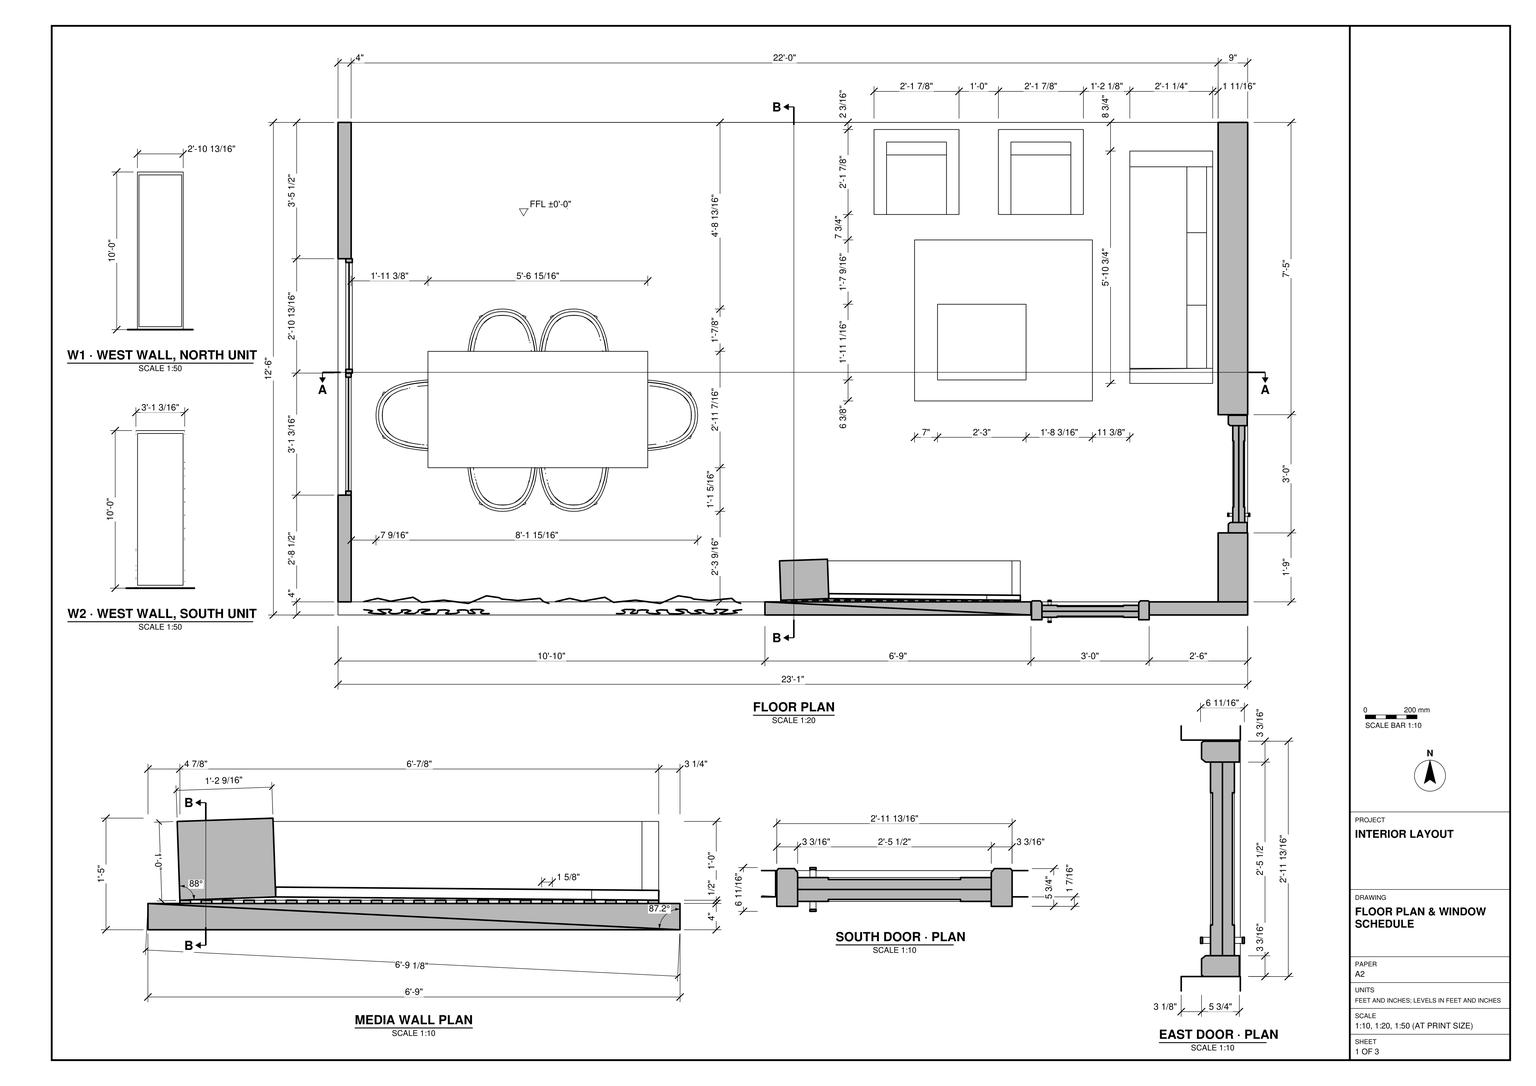
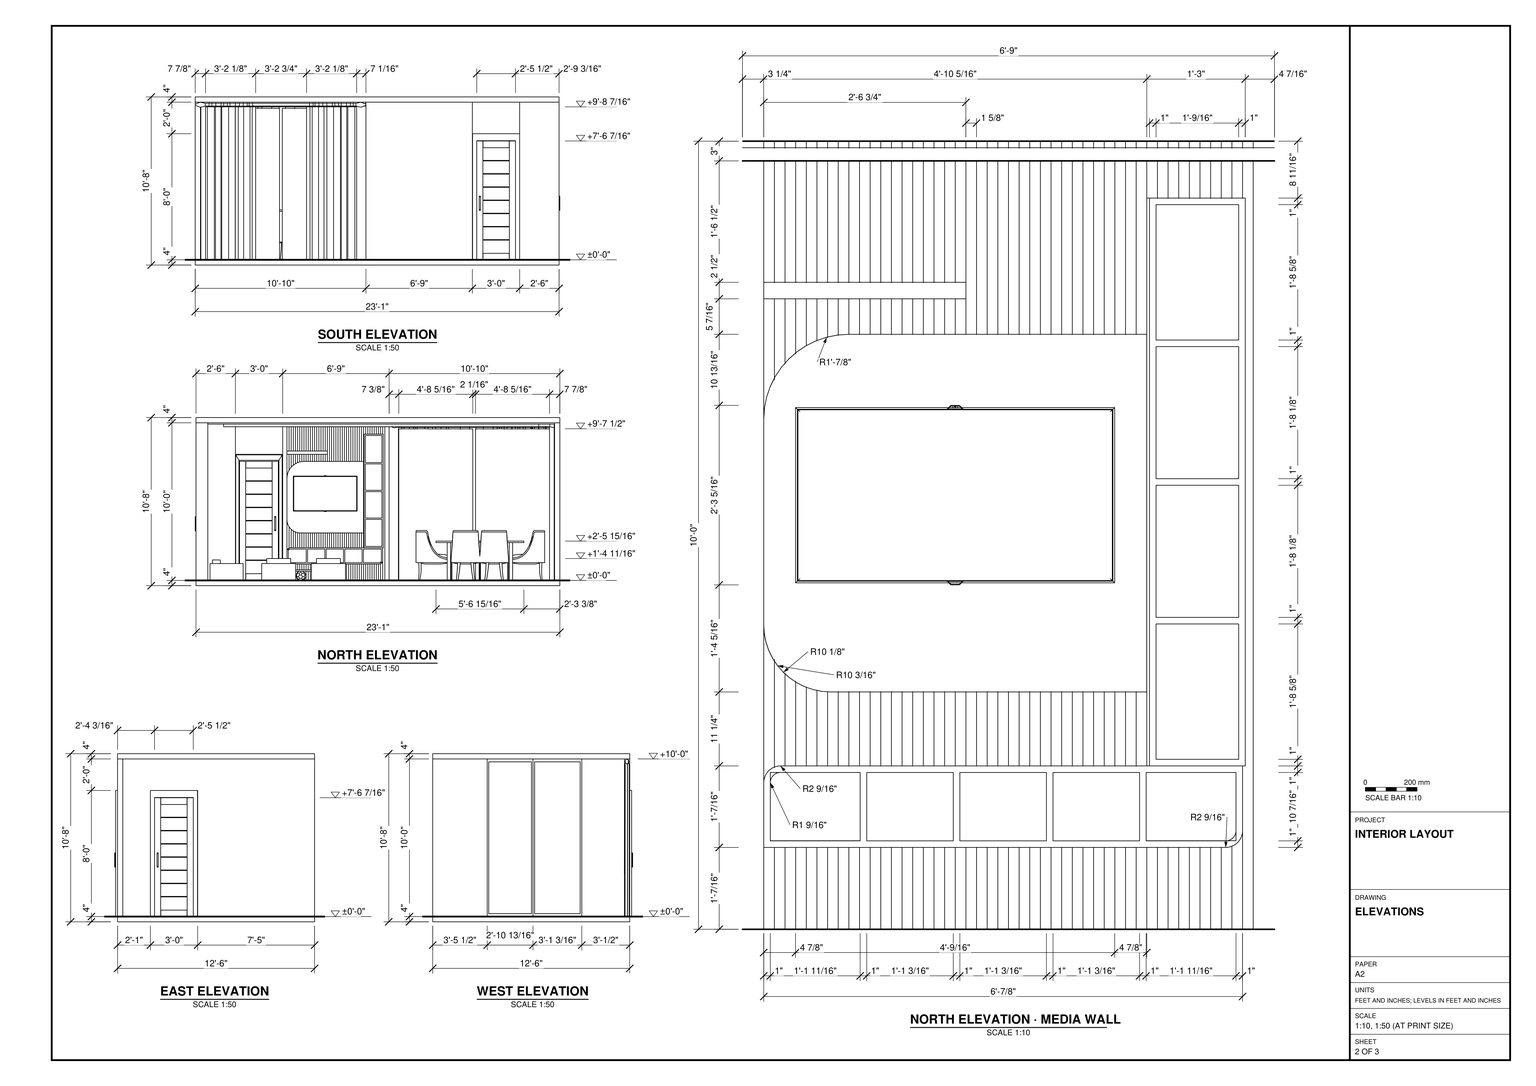
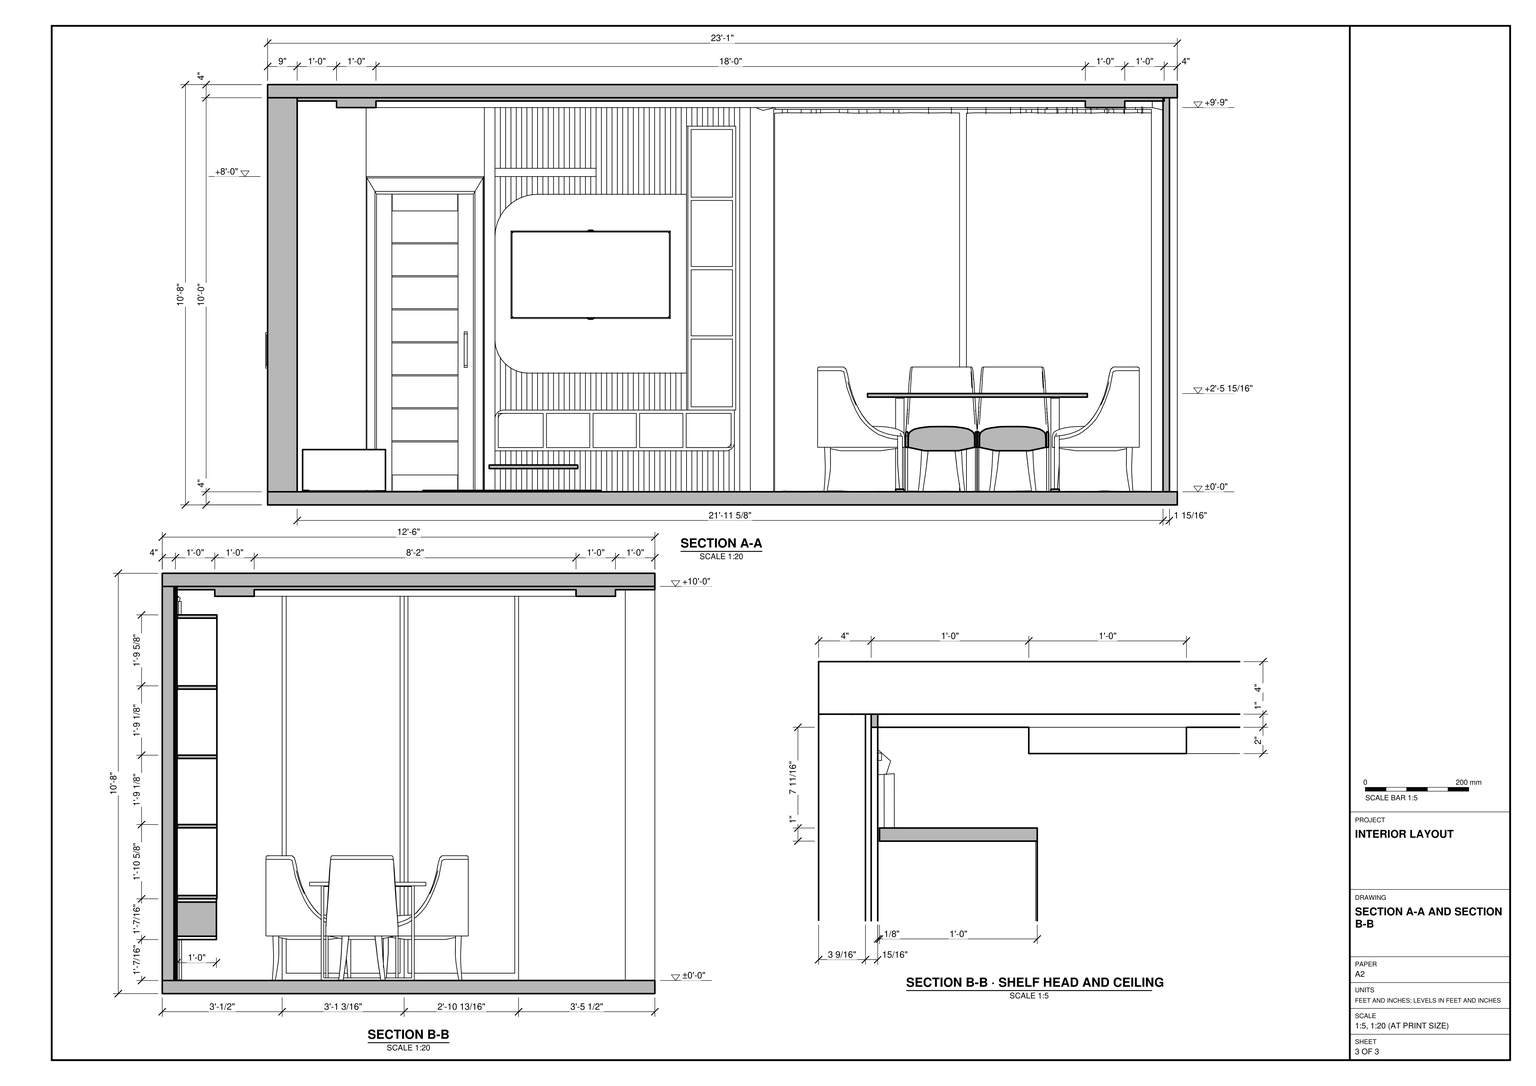
Build the living and dining interior in SketchUp from task_files/diagram_01.pdf. Work in feet and inches. Set the finished floor at ±0'-0" and make the overall model 23'-1 5/8" east to west, 12'-8 3/16" north to south and 10'-8" high.

Use the plan for the wall runs, thicknesses and opening positions. Model the floor and ceiling slabs and follow the sections for the stepped ceiling profile. Fit the two full-height window units in the west wall, place the framed doors near the southeast corner in their respective walls, and include the curtained opening along the south side of the dining area.

Place the rectangular dining table and six chairs at the west end. At the east end, arrange the sofa, two armchairs and low table around the rug as drawn. Build the media wall along the south side between the dining area and the south door. Follow its shallow angled profile in plan and use the enlarged elevation for the vertical slats, rounded screen backing, television, shelf, low storage bays and tall shelving at the dining end.

Keep the shell elements and each furniture or joinery piece in separate groups or components, and use components for repeated parts. Decor and loose items such as the rug and curtains may be any suitable library components. Save one SketchUp model as output_files/furnished_living_and_dining_room_with_a_media_wall.skp.

# SketchUp Ruby script. Lengths in inches.
U = 1.inch
M = Sketchup.active_model
def pt(a) = Geom::Point3d.new(a.map { |v| v * U })
def face(e, loops, mat)
  f = e.add_face(loops[0].map { |a| pt(a) })
  loops[1..].each { |l| e.add_face(l.map { |a| pt(a) }).erase! }
  f.material = f.back_material = mat if mat
  f
end
# faces: each face lists its corners as indices into pts; further lists are holes
def faces(e, pts, list, mat = nil) = list.each { |f| face(e, (f[0].is_a?(Array) ? f : [f]).map { |l| l.map { |i| pts[i] } }, mat) }
# xy, xz, yz: faces in a plane at the given z, y or x. An outline is a flat list of corners, or four numbers for a rectangle; further outlines are holes
def ring(l) = l.size == 4 ? [[l[0], l[1]], [l[2], l[1]], [l[2], l[3]], [l[0], l[3]]] : l.each_slice(2).to_a
def flat(e, list, mat, &to3) = list.each { |f| face(e, (f[0].is_a?(Array) ? f : [f]).map { |l| ring(l).map { |u, v| to3.(u, v) } }, mat) }
def xy(e, z, list, mat = nil) = flat(e, list, mat) { |x, y| [x, y, z] }
def xz(e, y, list, mat = nil) = flat(e, list, mat) { |x, z| [x, y, z] }
def yz(e, x, list, mat = nil) = flat(e, list, mat) { |y, z| [x, y, z] }
def lines(e, pts, list) = list.each { |a, b| e.add_line(pt(pts[a]), pt(pts[b])) }
# prism: a flat outline (further loops are holes) pulled along v
def prism(e, loops, v, mat = nil)
  f = face(e, loops, mat); d = Geom::Vector3d.new(v.map { |x| x * U })
  f.pushpull(f.normal.samedirection?(d) ? d.length : -d.length)
end
def box(e, o, s, mat = nil) = prism(e, [[o, [o[0] + s[0], o[1], o[2]], [o[0] + s[0], o[1] + s[1], o[2]], [o[0], o[1] + s[1], o[2]]]], [0, 0, s[2]], mat)
def at(x, y, z, deg = 0) = Geom::Transformation.translation(pt([x, y, z])) * Geom::Transformation.rotation(ORIGIN, Z_AXIS, deg.degrees)
def axes(o, x, y, z) = Geom::Transformation.new([*x, 0, *y, 0, *z, 0, *pt(o).to_a, 1])
def part(name) = M.definitions.add(name)
# library, detail: a bought-in or finely detailed component or shape, given as its bounding box
def library(name, o, s) = part(name).tap { |d| box(d.entities, o, s) }
def detail(e, o, s) = box(e.add_group.entities, o, s)
def put(e, d, t, mat = nil) = e.add_instance(d, t).tap { |i| i.material = mat if mat }
def group(e, t, mat = nil) = e.add_group.tap { |g| g.transformation = t; g.material = mat if mat }.entities
root = M.entities
M.materials.add("Carpete_com_padrão_de_quadrados_folheados_cor_de_canela").color = [77, 77, 77]
M.materials.add("Cor_008").color = [30, 30, 30]
M.materials.add("Cor_B05").color = [255, 243, 239]
M.materials.add("Emissive").color = [247, 235, 155]
M.materials.add("[Carpet_Berber_Multi]1").color = [151, 134, 121]
M.materials.add("[Color M07]").color = [58, 58, 58]
M.materials.add("[Stone Brushed Khaki]").color = [226, 197, 133]
M.materials.add("[Stone Vein Gray]").color = [166, 165, 165]
M.materials.add("[Translucent Glass Gray]3").color = [128, 128, 128]
M.materials["[Translucent Glass Gray]3"].alpha = 0.3
M.materials.add("[Translucent Glass Sky Reflection]").color = [126, 138, 183]
M.materials["[Translucent Glass Sky Reflection]"].alpha = 0.52
M.materials.add("[Wood Bamboo]").color = [177, 105, 43]
c1 = library("元件\#5",[-4.39,0,0],[5.37,35.83,90.55])
c2 = part("WINDOW (1)")
xy(c2.entities,0,[[0,0,59.06,1.97]],"[Color M07]")
xy(c2.entities,1.97,[[1.97,0,57.09,0.98],[1.97,0.98,57.09,1.97]],"[Color M07]")
xy(c2.entities,104.33,[[1.97,0,57.09,0.98],[1.97,0.98,57.09,1.97]],"[Color M07]")
xy(c2.entities,106.3,[[0,0,59.06,1.97]],"[Color M07]")
xz(c2.entities,0,[[[0,0,59.06,106.3],[1.97,1.97,57.09,104.33]]],"[Color M07]")
xz(c2.entities,0.98,[[1.97,1.97,57.09,104.33]],"[Translucent Glass Gray]3")
xz(c2.entities,1.97,[[[0,0,59.06,106.3],[1.97,1.97,57.09,104.33]]],"[Color M07]")
yz(c2.entities,0,[[0,0,1.97,106.3]],"[Color M07]")
yz(c2.entities,1.97,[[0,1.97,0.98,104.33],[0.98,1.97,1.97,104.33]],"[Color M07]")
yz(c2.entities,57.09,[[0,1.97,0.98,104.33],[0.98,1.97,1.97,104.33]],"[Color M07]")
yz(c2.entities,59.06,[[0,0,1.97,106.3]],"[Color M07]")
c3 = library("шторы раздвинутые\#1",[23.6875,-79.37,-3.6],[68.3125,79.85,10.87])
c4 = part("Buckyball")
xy(c4.entities,0,[[-8.55,-19.21,-14.73,-8.51,-20.91,2.2,-12.64,11.38,-4.37,20.57,18.21,10.51,15.63,-14.07]])
xy(c4.entities,115.07,[[4.37,-20.57,12.64,-11.38,20.91,-2.2,14.73,8.51,8.55,19.21,-15.63,14.07,-18.21,-10.51]])
p = [[3.54,-16.64,0],[15.63,-14.07,0],[31.26,-28.14,13],[22.7,-47.35,25.99],[-1.48,-52.49,25.99],[-17.11,-38.42,13],
  [-8.55,-19.21,0],[-38.02,-36.22,25.99],[-50.38,-14.81,25.99],[-41.83,4.4,13],[-20.91,2.2,0],[-14.73,-8.51,0],
  [52.05,6.96,25.99],[49.47,-17.63,25.99],[16.92,-1.78,0],[18.21,10.51,0],[36.42,21.03,13],[-8.74,41.14,13],
  [-4.37,20.57,0],[-12.64,11.38,0],[-46.2,24.97,25.99],[-29.66,43.34,25.99],[9.47,51.65,25.99],[32.05,41.6,25.99],
  [6.92,15.54,0],[-12.73,-58.99,47.02],[-35.32,-48.9375,47.02],[52.17,-30.34,47.02],[35.63,-48.71,47.02],[-60.04,-6.12,47.02],
  [-57.46,18.47,47.02],[44.98,40.24,47.02],[57.34,18.83,47.02],[-24.37,55.21,47.02],[-0.19,60.35,47.02],[24.37,-55.21,68.05],
  [0.19,-60.35,68.05],[-44.98,-40.24,68.05],[-57.34,-18.83,68.05],[60.04,6.12,68.05],[57.46,-18.47,68.05],[-52.17,30.34,68.05],
  [-35.63,48.71,68.05],[12.73,58.99,68.05],[35.32,48.9375,68.05],[-9.47,-51.65,89.08],[-32.05,-41.6,89.08],[46.2,-24.97,89.08],
  [29.66,-43.34,89.08],[-52.05,-6.96,89.08],[-49.47,17.63,89.08],[38.02,36.22,89.08],[50.38,14.81,89.08],[-22.7,47.35,89.08],
  [1.48,52.49,89.08],[8.74,-41.14,102.08],[-36.42,-21.03,102.08],[41.83,-4.4,102.08],[-31.26,28.14,102.08],[17.11,38.42,102.08],
  [4.37,-20.57,115.07],[-6.92,-15.54,115.07],[-18.21,-10.51,115.07],[20.91,-2.2,115.07],[12.64,-11.38,115.07],[-16.92,1.78,115.07],
  [-15.63,14.07,115.07],[8.55,19.21,115.07],[14.73,8.51,115.07],[-3.54,16.64,115.07]]
faces(c4.entities,p,[[0,1,2,3,4,5,6],[7,8,9,10,11,6,5],[12,13,2,1,14,15,16],[17,18,19,10,9,20,21],[22,23,16,15,24,18,17],[4,25,26,7,5],[13,27,28,3,2],[8,29,30,20,9],
  [23,31,32,12,16],[21,33,34,22,17],[3,28,35,36,25,4],[7,26,37,38,29,8],[12,32,39,40,27,13],[20,30,41,42,33,21],[22,34,43,44,31,23],[36,45,46,37,26,25],
  [40,47,48,35,28,27],[38,49,50,41,30,29],[44,51,52,39,32,31],[42,53,54,43,34,33],[35,48,55,45,36],[37,46,56,49,38],[39,52,57,47,40],[41,50,58,53,42],
  [43,54,59,51,44],[56,46,45,55,60,61,62],[57,63,64,60,55,48,47],[56,62,65,66,58,50,49],[59,67,68,63,57,52,51],[69,67,59,54,53,58,66]])
c5 = part("sofa+set1")
box(c5.entities,[-42.71,100.875,15.24],[52.75,61.75,2.5])
xy(c5.entities,0,[[-45.15,-29.2,-34.61,-24.95],[-34.61,-29.2,105.89,-24.95],[105.89,-29.2,116.85,28.55]])
xy(c5.entities,0,[[-57.35,54.63,54.9,178.63]],"Carpete_com_padrão_de_quadrados_folheados_cor_de_canela")
xy(c5.entities,14.5,[[-34.61,-24.95,-34.61,28.55,-35.18,28.55]])
xy(c5.entities,28.5,[[-45.15,-29.2,-45.15,28.55,-35.18,28.55,-34.61,-24.95,-34.61,-29.2],[-34.61,-29.2,105.89,-24.95],[105.89,-29.2,116.85,28.55],[72.64,60.92,72.64,69.66,123.16,69.66,123.16,111.4375,72.64,111.4375,72.64,120.17,131.89,120.17,131.89,60.92],[72.64,147.625,72.64,156.36,123.16,156.36,123.16,198.14,72.64,198.14,72.64,206.875,131.89,206.875,131.89,147.625]],"Cor_008")
xy(c5.entities,34.75,[[-34.61,-24.95,9.39,-11.2],[9.39,-24.95,59.96,-11.2],[59.96,-24.95,105.89,-11.2]],"[Carpet_Berber_Multi]1")
xy(c5.entities,37.25,[[114.17,69.66,123.16,111.4375],[114.17,156.36,123.16,198.14]],"[Carpet_Berber_Multi]1")
xz(c5.entities,-29.2,[[-45.15,0,-34.61,28.5],[-34.61,0,105.89,28.5],[105.89,0,116.85,28.5]],"Cor_008")
xz(c5.entities,-24.95,[[-34.61,28.5,105.89,34.75]])
xz(c5.entities,-11.2,[[-34.61,14.5,-30.99,15.1875,-27.34,15.75,-23.67,16.1875,-19.99,16.5,-16.3,16.6875,-12.61,16.75,-8.92,16.6875,-5.24,16.5,-1.56,16.1875,2.11,15.75,5.76,15.1875,9.39,14.5],[9.39,14.5,13.57,15.17,17.77,15.71,21.98,16.14,26.21,16.44,30.4375,16.625,34.67,16.6875,38.91,16.625,43.14,16.44,47.36,16.14,51.58,15.71,55.78,15.17,59.96,14.5]])
xz(c5.entities,-11.2,[[-34.61,14.5,-34.61,34.75,9.39,34.75,9.39,14.5,5.76,15.1875,2.11,15.75,-1.56,16.1875,-5.24,16.5,-8.92,16.6875,-12.61,16.75,-16.3,16.6875,-19.99,16.5,-23.67,16.1875,-27.34,15.75,-30.99,15.1875],[9.39,14.5,9.39,34.75,59.96,34.75,59.96,14.5,55.78,15.17,51.58,15.71,47.36,16.14,43.14,16.44,38.91,16.625,34.67,16.6875,30.4375,16.625,26.21,16.44,21.98,16.14,17.77,15.71,13.57,15.17],[59.96,14.5,63.75,15.17,67.5625,15.71,71.39,16.14,75.23,16.44,79.08,16.625,82.93,16.6875,86.77,16.625,90.62,16.44,94.46,16.14,98.29,15.71,102.1,15.17,105.89,14.5,105.89,34.75,59.96,34.75]],"[Carpet_Berber_Multi]1")
xz(c5.entities,28.55,[[-45.15,0,-35.18,28.5],[-35.18,0,105.89,7.25],[105.89,0,116.85,28.5]],"Cor_008")
xz(c5.entities,28.55,[[-35.18,7.25,-35.18,14.5,-34.61,14.5,-30.99,15.1875,-27.34,15.75,-23.67,16.1875,-19.99,16.5,-16.3,16.6875,-12.61,16.75,-8.92,16.6875,-5.24,16.5,-1.56,16.1875,2.11,15.75,5.76,15.1875,9.39,14.5,13.57,15.17,17.77,15.71,21.98,16.14,26.21,16.44,30.4375,16.625,34.67,16.6875,38.91,16.625,43.14,16.44,47.36,16.14,51.58,15.71,55.78,15.17,59.96,14.5,63.75,15.17,67.5625,15.71,71.39,16.14,75.23,16.44,79.08,16.625,82.93,16.6875,86.77,16.625,90.62,16.44,94.46,16.14,98.29,15.71,102.1,15.17,105.89,14.5,105.89,7.25]],"Cor_B05")
xz(c5.entities,60.92,[[72.64,0,131.89,28.5]])
xz(c5.entities,69.66,[[72.64,14.5,114.17,28.5]],"Cor_008")
xz(c5.entities,69.66,[[114.17,28.5,123.16,37.25]],"[Carpet_Berber_Multi]1")
xz(c5.entities,111.4375,[[72.64,14.5,114.17,28.5]])
xz(c5.entities,111.4375,[[114.17,28.5,123.16,37.25]],"[Carpet_Berber_Multi]1")
xz(c5.entities,120.17,[[72.64,0,131.89,28.5]],"Cor_008")
xz(c5.entities,147.625,[[72.64,0,131.89,28.5]])
xz(c5.entities,156.36,[[72.64,14.5,114.17,28.5]],"Cor_008")
xz(c5.entities,156.36,[[114.17,28.5,123.16,37.25]],"[Carpet_Berber_Multi]1")
xz(c5.entities,198.14,[[72.64,14.5,114.17,28.5]])
xz(c5.entities,198.14,[[114.17,28.5,123.16,37.25]],"[Carpet_Berber_Multi]1")
xz(c5.entities,206.875,[[72.64,0,131.89,28.5]],"Cor_008")
yz(c5.entities,-45.15,[[-29.2,0,28.55,28.5]],"Cor_008")
yz(c5.entities,-34.61,[[-29.2,14.5,-24.95,20.25],[-29.2,20.25,-24.95,28.5]])
yz(c5.entities,-34.61,[[-24.95,14.5,-11.2,34.75]],"[Carpet_Berber_Multi]1")
yz(c5.entities,72.64,[[69.66,0,111.4375,7.25],[156.36,0,198.14,7.25]])
yz(c5.entities,72.64,[[60.92,0,69.66,28.5],[111.4375,0,120.17,28.5],[147.625,0,156.36,28.5],[198.14,0,206.875,28.5]],"Cor_008")
yz(c5.entities,72.64,[[69.66,7.25,111.4375,7.25,111.4375,14.5,107.99,15.11,104.52,15.61,101.04,16,97.55,16.28,94.05,16.44,90.55,16.5,87.05,16.44,83.55,16.28,80.05,16,76.57,15.61,73.11,15.11,69.66,14.5],[156.36,7.25,198.14,7.25,198.14,14.5,194.7,15.1875,191.24,15.75,187.76,16.1875,184.26,16.5,180.76,16.6875,177.25,16.75,173.74,16.6875,170.24,16.5,166.74,16.1875,163.26,15.75,159.8,15.1875,156.36,14.5]],"Cor_B05")
yz(c5.entities,105.89,[[-11.2,14.5,28.55,28.5]],"Cor_008")
yz(c5.entities,105.89,[[-24.95,28.5,-11.2,34.75]],"[Carpet_Berber_Multi]1")
yz(c5.entities,114.17,[[69.66,14.5,73.11,15.11,76.57,15.61,80.05,16,83.55,16.28,87.05,16.44,90.55,16.5,94.05,16.44,97.55,16.28,101.04,16,104.52,15.61,107.99,15.11,111.4375,14.5,111.4375,37.25,69.66,37.25],[156.36,14.5,159.8,15.1875,163.26,15.75,166.74,16.1875,170.24,16.5,173.74,16.6875,177.25,16.75,180.76,16.6875,184.26,16.5,187.76,16.1875,191.24,15.75,194.7,15.1875,198.14,14.5,198.14,37.25,156.36,37.25]],"[Carpet_Berber_Multi]1")
yz(c5.entities,116.85,[[-29.2,0,28.55,28.5]],"Cor_008")
yz(c5.entities,123.16,[[69.66,28.5,111.4375,37.25],[156.36,28.5,198.14,37.25]],"[Carpet_Berber_Multi]1")
yz(c5.entities,131.89,[[60.92,0,120.17,28.5],[147.625,0,206.875,28.5]])
p = [[-35.18,28.55,28.5],[-35.18,28.55,14.5],[-34.61,-24.95,14.5],[-34.61,-24.95,20.25],[-34.61,-24.95,28.5],[-34.61,28.55,14.5],
  [-34.61,-11.2,14.5],[-30.99,-11.2,15.1875],[-30.99,28.55,15.1875],[5.76,28.55,15.1875],[5.76,-11.2,15.1875],[9.39,-11.2,14.5],
  [9.39,28.55,14.5],[13.57,28.55,15.17],[13.57,-11.2,15.17],[59.96,28.55,14.5],[55.78,28.55,15.17],[55.78,-11.2,15.17],
  [59.96,-11.2,14.5],[63.75,28.55,15.17],[63.75,-11.2,15.17],[105.89,28.55,14.5],[102.1,28.55,15.17],[102.1,-11.2,15.17],
  [105.89,-11.2,14.5],[72.64,69.66,14.5],[114.17,69.66,14.5],[114.17,73.11,15.11],[72.64,73.11,15.11],[114.17,107.99,15.11],
  [114.17,111.4375,14.5],[72.64,111.4375,14.5],[72.64,107.99,15.11],[72.64,156.36,14.5],[114.17,156.36,14.5],[114.17,159.8,15.1875],
  [72.64,159.8,15.1875],[114.17,194.7,15.1875],[114.17,198.14,14.5],[72.64,198.14,14.5],[72.64,194.7,15.1875],[114.17,76.57,15.61],
  [72.64,76.57,15.61],[114.17,104.52,15.61],[72.64,104.52,15.61],[-27.34,-11.2,15.75],[-27.34,28.55,15.75],[2.11,28.55,15.75],
  [2.11,-11.2,15.75],[17.77,28.55,15.71],[17.77,-11.2,15.71],[51.58,28.55,15.71],[51.58,-11.2,15.71],[67.5625,28.55,15.71],
  [67.5625,-11.2,15.71],[98.29,28.55,15.71],[98.29,-11.2,15.71],[114.17,163.26,15.75],[72.64,163.26,15.75],[114.17,191.24,15.75],
  [72.64,191.24,15.75],[114.17,80.05,16],[72.64,80.05,16],[114.17,101.04,16],[72.64,101.04,16],[-23.67,-11.2,16.1875],
  [-23.67,28.55,16.1875],[-1.56,28.55,16.1875],[-1.56,-11.2,16.1875],[21.98,28.55,16.14],[21.98,-11.2,16.14],[47.36,28.55,16.14],
  [47.36,-11.2,16.14],[71.39,28.55,16.14],[71.39,-11.2,16.14],[94.46,28.55,16.14],[94.46,-11.2,16.14],[114.17,166.74,16.1875],
  [72.64,166.74,16.1875],[114.17,187.76,16.1875],[72.64,187.76,16.1875],[114.17,83.55,16.28],[72.64,83.55,16.28],[114.17,97.55,16.28],
  [72.64,97.55,16.28],[26.21,28.55,16.44],[26.21,-11.2,16.44],[43.14,28.55,16.44],[43.14,-11.2,16.44],[75.23,28.55,16.44],
  [75.23,-11.2,16.44],[90.62,28.55,16.44],[90.62,-11.2,16.44],[-19.99,-11.2,16.5],[-19.99,28.55,16.5],[-5.24,28.55,16.5],
  [-5.24,-11.2,16.5],[114.17,170.24,16.5],[72.64,170.24,16.5],[114.17,184.26,16.5],[72.64,184.26,16.5],[114.17,87.05,16.44],
  [72.64,87.05,16.44],[114.17,94.05,16.44],[72.64,94.05,16.44],[30.4375,28.55,16.625],[30.4375,-11.2,16.625],[38.91,28.55,16.625],
  [38.91,-11.2,16.625],[79.08,28.55,16.625],[79.08,-11.2,16.625],[86.77,28.55,16.625],[86.77,-11.2,16.625],[114.17,90.55,16.5],
  [72.64,90.55,16.5],[-16.3,-11.2,16.6875],[-16.3,28.55,16.6875],[-8.92,28.55,16.6875],[-8.92,-11.2,16.6875],[114.17,173.74,16.6875],
  [72.64,173.74,16.6875],[114.17,180.76,16.6875],[72.64,180.76,16.6875],[34.67,28.55,16.6875],[34.67,-11.2,16.6875],[82.93,28.55,16.6875],
  [82.93,-11.2,16.6875],[-12.61,-11.2,16.75],[-12.61,28.55,16.75],[114.17,177.25,16.75],[72.64,177.25,16.75]]
faces(c5.entities,p,[[0,1,2,3,4]],"Cor_008")
faces(c5.entities,p,[[5,6,7,8],[9,10,11,12],[13,12,11,14],[15,16,17,18],[19,15,18,20],[21,22,23,24],[25,26,27,28],[29,30,31,32],
  [33,34,35,36],[37,38,39,40],[28,27,41,42],[43,29,32,44],[8,7,45,46],[47,48,10,9],[49,13,14,50],[16,51,52,17],
  [53,19,20,54],[22,55,56,23],[36,35,57,58],[59,37,40,60],[42,41,61,62],[63,43,44,64],[46,45,65,66],[67,68,48,47],
  [69,49,50,70],[51,71,72,52],[73,53,54,74],[55,75,76,56],[58,57,77,78],[79,59,60,80],[62,61,81,82],[83,63,64,84],
  [85,69,70,86],[71,87,88,72],[89,73,74,90],[75,91,92,76],[66,65,93,94],[95,96,68,67],[78,77,97,98],[99,79,80,100],
  [82,81,101,102],[103,83,84,104],[105,85,86,106],[87,107,108,88],[109,89,90,110],[91,111,112,92],[102,101,113,114],[113,103,104,114],
  [94,93,115,116],[117,118,96,95],[98,97,119,120],[121,99,100,122],[123,105,106,124],[107,123,124,108],[125,109,110,126],[111,125,126,112],
  [116,115,127,128],[128,127,118,117],[120,119,129,130],[129,121,122,130]],"Cor_B05")
lines(c5.entities,p,[[24,18],[34,38],[26,30]])
put(c5.entities,c4,axes([-12.625,129.36,-0.92],[0.14052,0,0],[0,0.14052,0],[0,0,0.14052]))
c6 = library("Dining set",[0,0,0],[61.62,97.96,38])
c7 = library("download?mid=50c7180b9fccec56d493bfe20f94b6ab&ctyp=sp&cv=p8.",[149.43,43.83,17.86],[74.75,0.57,42.04])
c8 = library("Group\#3",[0,0,0],[117,4.5,120])
c9 = library("Group\#7",[0,0,0],[72.9,12,12.41])
xy(root,50.49,[[135.8,7.17,148.44,8.53]],"Emissive")
xy(root,71.61,[[135.86,6.74,148.42,7.91]],"Emissive")
xy(root,92.72,[[135.79,7.17,148.44,8.9]],"Emissive")
xy(root,100,[[176.98,6.71,207.76,8.19]],"Emissive")
xy(root,114.33,[[135.79,7.17,148.44,8.73]],"Emissive")
xy(root,121,[[[16,18.21,256,140.21],[28,30.21,244,128.21]]])
xy(root,123,[[[4,6.21,268,152.21],[16,18.21,256,140.21]],[28,30.21,244,128.21]])
xy(root,124,[[4,6.21,268,152.21]])
xz(root,6.21,[[4,123,268,124]])
xz(root,18.21,[[16,121,256,123]])
xz(root,18.7,[[150.54,17.47,163.72,27.88],[164.72,17.47,177.9,27.88],[178.9,17.47,192.08,27.88],[135.86,17.48,149.54,27.88],[193.08,17.49,206.76,27.88]],"[Translucent Glass Sky Reflection]")
xz(root,30.21,[[28,121,244,123]],"Emissive")
xz(root,128.21,[[28,121,244,123]])
xz(root,140.21,[[16,121,256,123]],"Emissive")
xz(root,152.21,[[4,123,268,124]])
yz(root,4,[[6.21,123,152.21,124]])
yz(root,16,[[18.21,121,140.21,123]],"Emissive")
yz(root,28,[[30.21,121,128.21,123]],"Emissive")
yz(root,244,[[30.21,121,128.21,123]],"Emissive")
yz(root,256,[[18.21,121,140.21,123]],"Emissive")
yz(root,268,[[6.21,123,152.21,124]])
p = [[135.45,18.74,29.88],[135.45,18.74,50.49],[148.03,19.17,50.49],[148.03,19.17,29.88],[135.45,18.74,51.49],[135.45,18.74,71.61],
  [148.03,19.17,71.61],[148.03,19.17,51.49],[135.45,18.74,92.72],[148.03,19.17,92.72],[148.03,19.17,72.61],[135.45,18.74,72.61],
  [135.45,18.74,114.33],[148.03,19.17,114.33],[148.03,19.17,93.72],[135.45,18.74,93.72]]
faces(root,p,[[0,1,2,3],[4,5,6,7],[8,9,10,11],[12,13,14,15]],"[Translucent Glass Sky Reflection]")
put(root,c1,axes([276.39,27.21,4],[1.24,0,0],[0,1,0],[0,0,1.06017]))
put(root,c1,axes([211.17,1.22,4],[0,-1.24,0],[1,0,0],[0,0,1.06017]))
put(root,c2,axes([2.38,110.71,4],[0,-0.59,0],[1,0,0],[0,0,1.12889]))
put(root,c2,axes([2.38,75.87,4],[0,-0.6292,0],[0.82447,0,0],[0,0,1.12889]))
put(root,c3,axes([-45.08,8.73,123.28],[1.90307,0,0],[0,0,1.50293],[0,-1,0]))
put(root,c5,axes([253.58,92.44,4.4],[0,0.4368,0],[-0.4368,0,0],[0,0,0.4368]))
put(root,c6,at(109.52,33.77,4,90))
put(root,c7,axes([300.04,37.57,44.83],[-0.65,0,0],[0,-0.65,0],[0,0,0.65]))
g1 = group(root,at(0,6.21,0),"[Stone Vein Gray]")
box(g1,[0,-4,0],[277,150,4])
g2 = group(root,at(0,2.21,4))
prism(g2,[[[4,108.5,0],[0,108.5,0],[0,150,0],[4,150,0],[4,141,0]]],[0,0,120])
xy(g2,0,[[0,0,130,4],[211,0,247,4],[0,4,4,36.5],[268,4,277,25],[268,61,277,150]])
xy(g2,96,[[268,25,277,61]])
xy(g2,120,[[130,0,211,4],[247,0,277,4],[0,4,4,36.5],[268,4,277,150]])
xz(g2,0,[[130,0,211,120],[247,0,277,120]])
xz(g2,4,[[0,0,4,120],[130,0,211,120],[247,0,268,120],[268,0,277,120]])
xz(g2,25,[[268,0,277,96]])
xz(g2,36.5,[[0,0,4,120]])
xz(g2,61,[[268,0,277,96]])
xz(g2,150,[[268,0,277,120]])
yz(g2,0,[[4,0,36.5,120]])
yz(g2,4,[[4,0,36.5,120]])
yz(g2,130,[[0,0,4,120]])
yz(g2,211,[[0,0,4,120]])
yz(g2,247,[[0,0,4,120]])
yz(g2,268,[[4,0,4,120,150,120,150,0,61,0,61,96,25,96,25,0]])
yz(g2,277,[[0,0,4,120],[4,0,25,0,25,96,61,96,61,0,150,0,150,120,4,120]])
p = [[0,36.5,0],[0,108.5,0]]
lines(g2,p,[[0,1]])
put(root,c8,at(130,2.21,4))
g3 = group(root,at(134.45,6.71,28.88),"[Wood Bamboo]")
prism(g3,[[[14.99,0.5,0],[14.99,0.5,86.46],[0.41,0,86.46],[0.41,0,0]],[[1.41,0.03,64.84],[1.41,0.03,85.46],[13.99,0.47,85.46],[13.99,0.47,64.84]],[[13.99,0.47,21.61],[13.99,0.47,1],[1.41,0.03,1],[1.41,0.03,21.61]],[[13.99,0.47,22.61],[1.41,0.03,22.61],[1.41,0.03,42.73],[13.99,0.47,42.73]],[[13.99,0.47,43.73],[1.41,0.03,43.73],[1.41,0.03,63.84],[13.99,0.47,63.84]]],[-0.41,11.99,0])
g4 = group(root,at(149.44,6.71,40.14),"[Stone Brushed Khaki]")
xy(g4,0,[[48.1,0.09,0,0.5,0.01,2,48.12,1.59]],"Emissive")
xy(g4,54.46,[[45.4,0.11,45.41,1.61,0.01,2,0,0.5]],"Emissive")
p = [[58.32,0,10.22],[58.32,0,41.53],[58.21,0,43.22],[57.88,0,44.88],[57.34,0.01,46.48],[56.59,0.01,47.99],
  [55.65,0.02,49.4],[54.54,0.03,50.67],[53.26,0.04,51.78],[51.86,0.06,52.72],[50.34,0.07,53.47],[48.74,0.08,54.01],
  [47.08,0.1,54.34],[45.4,0.11,54.46],[0,0.5,54.46],[0,0.5,0],[48.1,0.09,0],[49.4375,0.08,0.09],
  [50.75,0.06,0.35],[52.01,0.05,0.78],[53.21,0.04,1.37],[54.32,0.03,2.11],[55.33,0.03,2.99],[56.21,0.02,4],
  [56.95,0.01,5.11],[57.54,0.01,6.31],[57.97,0,7.57],[58.23,0,8.88],[48.12,1.59,0],[49.45,1.58,0.09],
  [0.01,2,54.46],[0.01,2,0],[58.33,1.5,41.53],[58.33,1.5,10.22],[58.25,1.5,8.88],[57.98,1.5,7.57],
  [57.56,1.51,6.31],[56.96,1.51,5.11],[56.22,1.52,4],[55.34,1.53,2.99],[54.34,1.53,2.11],[53.23,1.54,1.37],
  [52.03,1.55,0.78],[50.76,1.56,0.35],[45.41,1.61,54.46],[47.1,1.6,54.34],[48.76,1.58,54.01],[50.36,1.57,53.47],
  [51.87,1.56,52.72],[53.28,1.54,51.78],[54.55,1.53,50.67],[55.66,1.52,49.4],[56.6,1.51,47.99],[57.35,1.51,46.48],
  [57.89,1.5,44.88],[58.22,1.5,43.22]]
faces(g4,p,[[0,1,2,3,4,5,6,7,8,9,10,11,12,13,14,15,16,17,18,19,20,21,22,23,24,25,26,27],[15,14,30,31],[32,33,34,35,36,37,38,39,40,41,42,43,29,28,31,30,44,45,46,47,48,49,50,51,52,53,54,55]])
faces(g4,p,[[17,16,28,29],[18,17,29,43],[19,18,43,42],[20,19,42,41],[21,20,41,40],[22,21,40,39],[23,22,39,38],[24,23,38,37],
  [25,24,37,36],[26,25,36,35],[27,26,35,34],[0,27,34,33],[1,0,33,32],[2,1,32,55],[3,2,55,54],[4,3,54,53],
  [5,4,53,52],[6,5,52,51],[7,6,51,50],[8,7,50,49],[9,8,49,48],[10,9,48,47],[11,10,47,46],[12,11,46,45],
  [13,12,45,44]],"Emissive")
g5 = group(root,at(176.98,6.71,100),"[Wood Bamboo]")
box(g5,[0,0,0],[30.78,12.46,2.51])
put(root,c9,at(134.86,6.7,16.47),"[Wood Bamboo]")
g6 = group(root,at(0,2.21,124))
box(g6,[0,0,0],[277,150,4])
